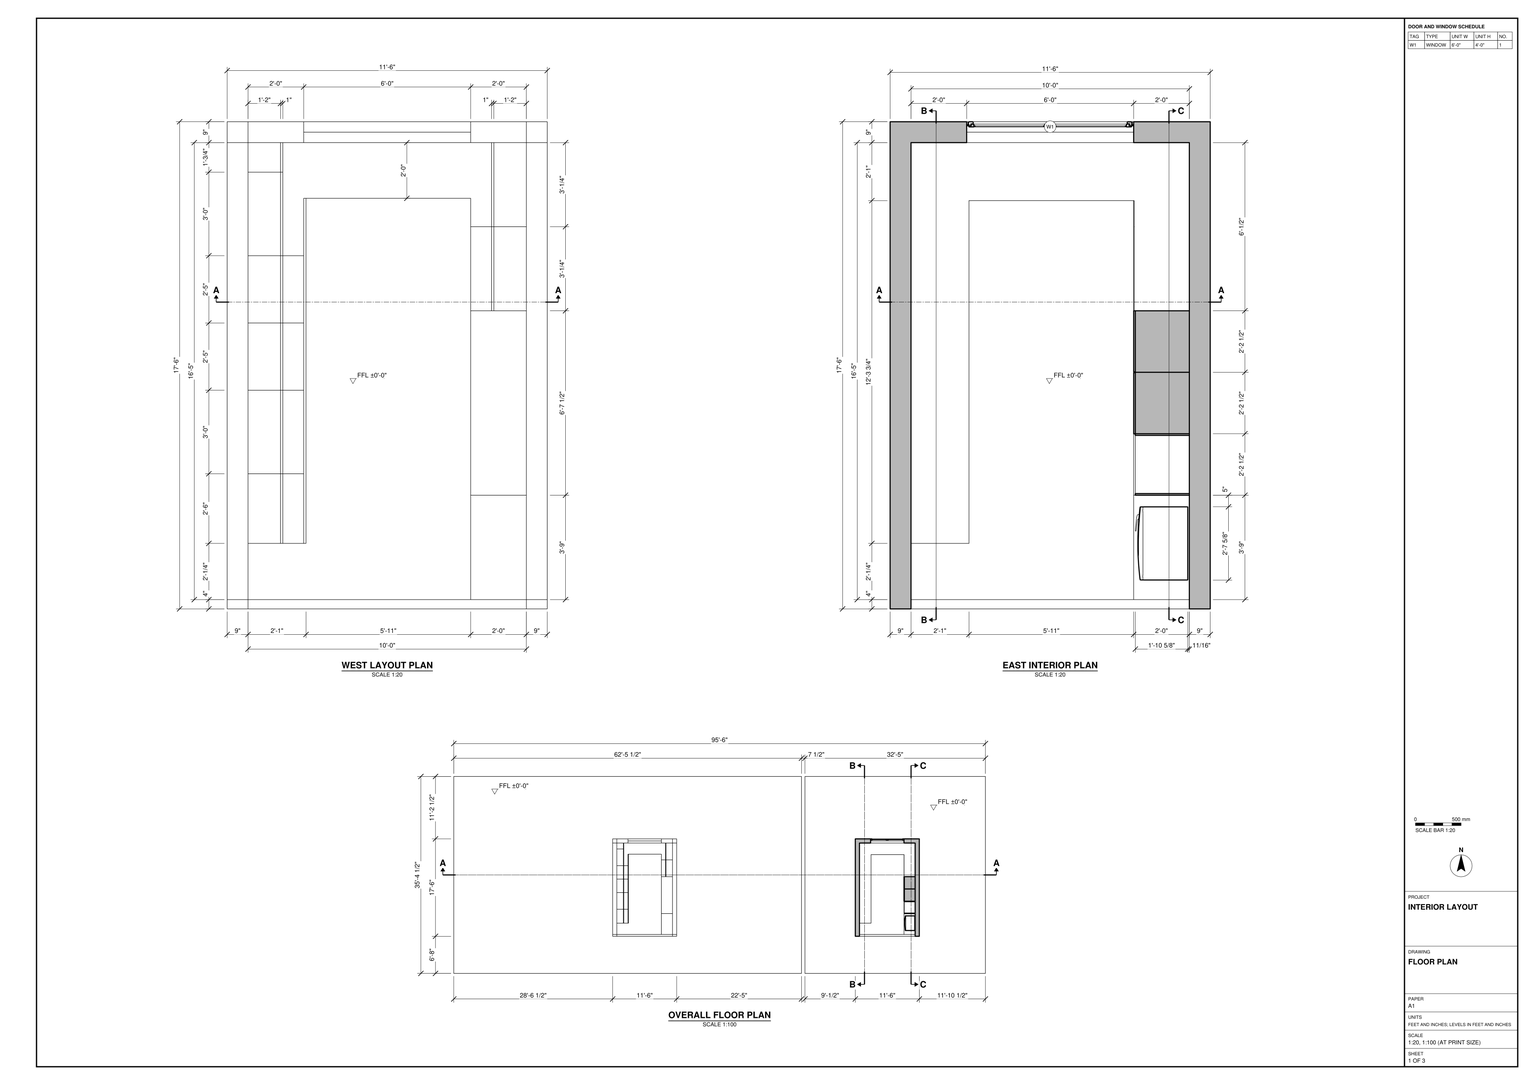
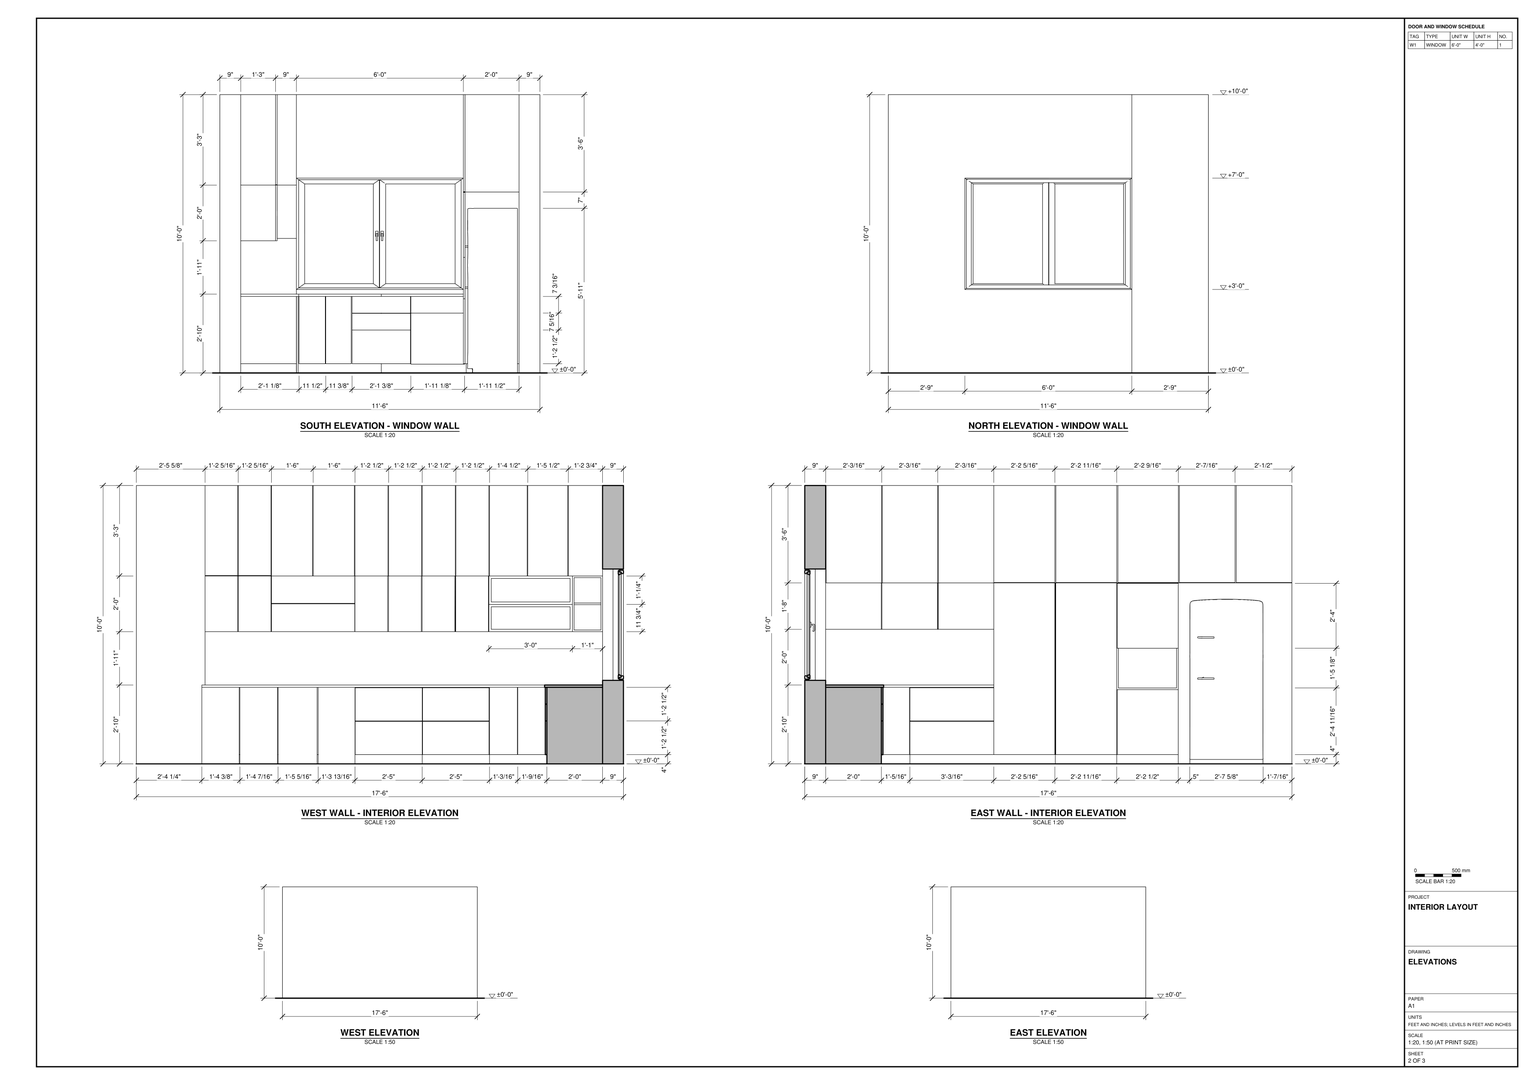
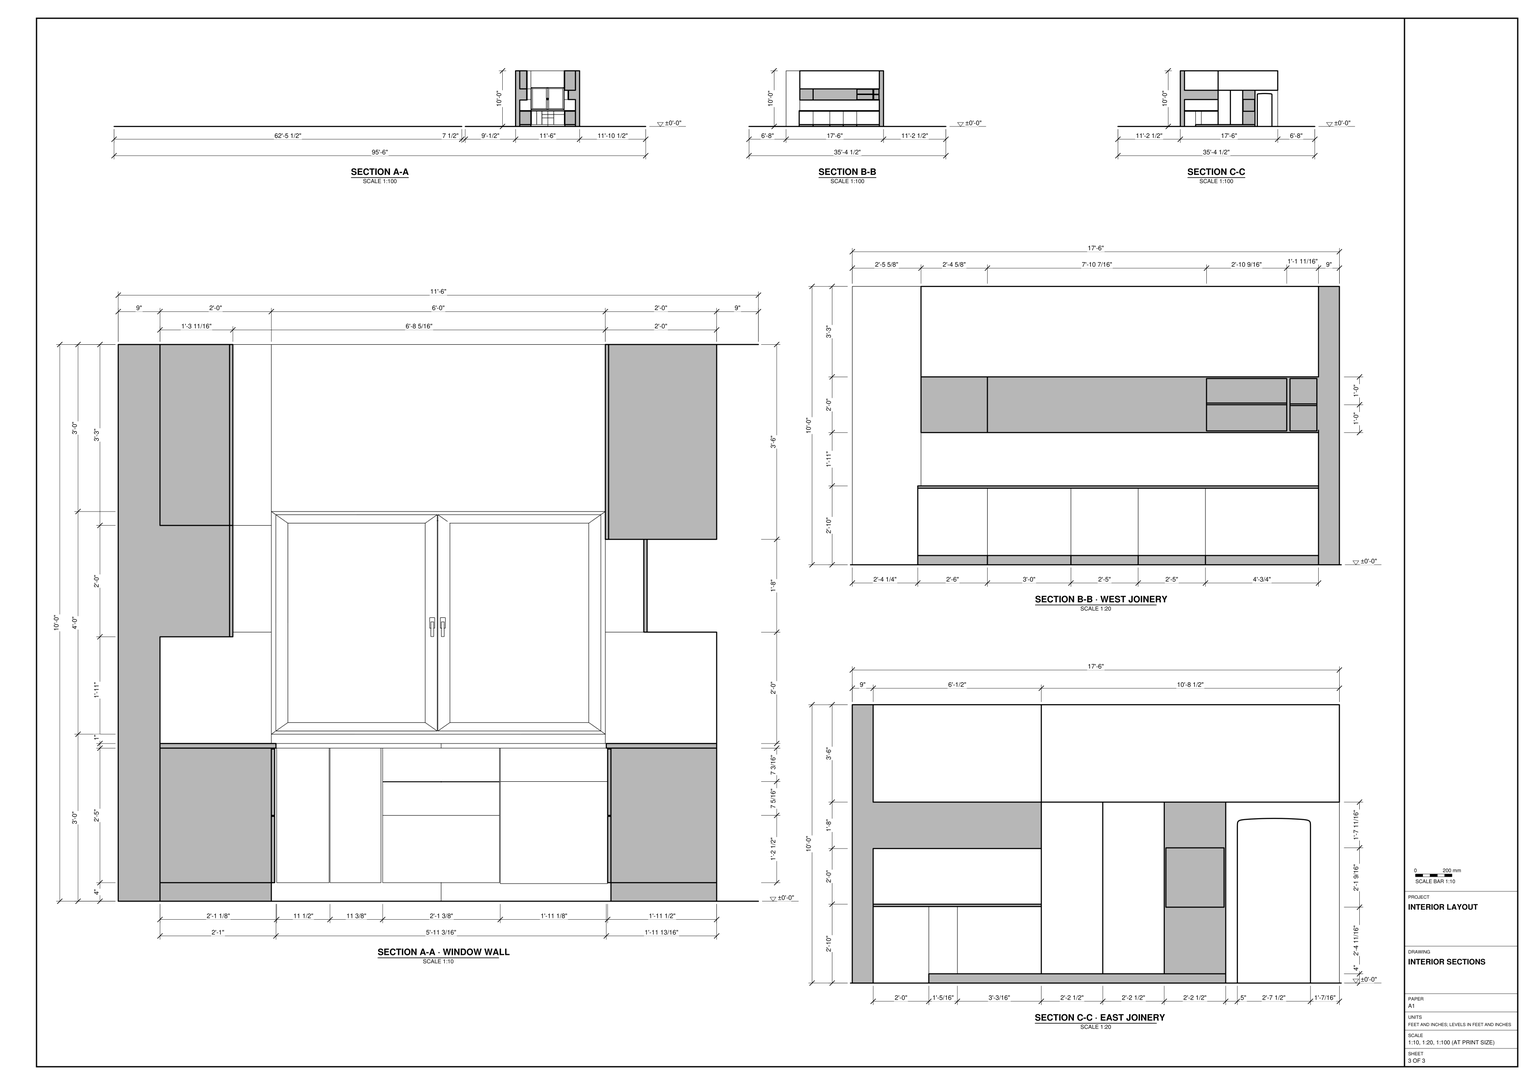
Build one SketchUp model from task_files/diagram_01.pdf. Work in feet and inches. The overall model measures 95'-6" along X, 35'-4 1/2" along Y and 10'-0" high, with a single finished floor level at ±0'-0".

Use the overall floor plan to position the two rectangular floor areas and the gap between them. Show the west layout as a flat plan with the wall outlines, cabinet divisions and central aisle. On the east floor area, build the corresponding kitchen in three dimensions. Its outside footprint is 11'-6" by 17'-6". Build the 9" side walls and window wall, leaving the entrance end open. Center the two-panel window above the counter on the end wall.

Use the interior elevations for the arrangement of cupboard doors, drawers and shelves, and the sections for worktop heights, plinths and cabinet depths. Connect the long west worktop to the base units beneath the window and the shorter east worktop. Continue the east run with tall storage and the refrigerator bay toward the entrance. Decor and loose items, including the refrigerator, may be any suitable library components.

Keep shell elements such as walls and floor areas, and each furniture or joinery piece, in separate groups or components. Use components for repeated parts. Save the completed model as output_files/fitted_kitchen_and_its_companion_plan_layout.skp.

# SketchUp Ruby script. Lengths in inches.
U = 1.inch
M = Sketchup.active_model
def pt(a) = Geom::Point3d.new(a.map { |v| v * U })
def face(e, loops, mat)
  f = e.add_face(loops[0].map { |a| pt(a) })
  loops[1..].each { |l| e.add_face(l.map { |a| pt(a) }).erase! }
  f.material = f.back_material = mat if mat
  f
end
# faces: each face lists its corners as indices into pts; further lists are holes
def faces(e, pts, list, mat = nil) = list.each { |f| face(e, (f[0].is_a?(Array) ? f : [f]).map { |l| l.map { |i| pts[i] } }, mat) }
# xy, xz, yz: faces in a plane at the given z, y or x. An outline is a flat list of corners, or four numbers for a rectangle; further outlines are holes
def ring(l) = l.size == 4 ? [[l[0], l[1]], [l[2], l[1]], [l[2], l[3]], [l[0], l[3]]] : l.each_slice(2).to_a
def flat(e, list, mat, &to3) = list.each { |f| face(e, (f[0].is_a?(Array) ? f : [f]).map { |l| ring(l).map { |u, v| to3.(u, v) } }, mat) }
def xy(e, z, list, mat = nil) = flat(e, list, mat) { |x, y| [x, y, z] }
def xz(e, y, list, mat = nil) = flat(e, list, mat) { |x, z| [x, y, z] }
def yz(e, x, list, mat = nil) = flat(e, list, mat) { |y, z| [x, y, z] }
def lines(e, pts, list) = list.each { |a, b| e.add_line(pt(pts[a]), pt(pts[b])) }
# prism: a flat outline (further loops are holes) pulled along v
def prism(e, loops, v, mat = nil)
  f = face(e, loops, mat); d = Geom::Vector3d.new(v.map { |x| x * U })
  f.pushpull(f.normal.samedirection?(d) ? d.length : -d.length)
end
def box(e, o, s, mat = nil) = prism(e, [[o, [o[0] + s[0], o[1], o[2]], [o[0] + s[0], o[1] + s[1], o[2]], [o[0], o[1] + s[1], o[2]]]], [0, 0, s[2]], mat)
def at(x, y, z, deg = 0) = Geom::Transformation.translation(pt([x, y, z])) * Geom::Transformation.rotation(ORIGIN, Z_AXIS, deg.degrees)
def axes(o, x, y, z) = Geom::Transformation.new([*x, 0, *y, 0, *z, 0, *pt(o).to_a, 1])
def part(name) = M.definitions.add(name)
# library, detail: a bought-in or finely detailed component or shape, given as its bounding box
def library(name, o, s) = part(name).tap { |d| box(d.entities, o, s) }
def detail(e, o, s) = box(e.add_group.entities, o, s)
def put(e, d, t, mat = nil) = e.add_instance(d, t).tap { |i| i.material = mat if mat }
def group(e, t, mat = nil) = e.add_group.tap { |g| g.transformation = t; g.material = mat if mat }.entities
root = M.entities
M.materials.add("Heather_Band").color = [201, 178, 162]
M.materials.add("[Basic Tile]").color = [203, 206, 202]
M.materials.add("[Color B01]").color = [255, 216, 204]
M.materials.add("[Color M00]").color = [255, 255, 255]
M.materials.add("[Marble Carrara Gold Floor Tile]").color = [225, 223, 217]
M.materials.add("[Translucent Glass Gray]").color = [128, 128, 128]
M.materials["[Translucent Glass Gray]"].alpha = 0.5
c1 = library("Fridge 143 008",[-15.8,-16.72,0],[31.6,33.44,70.99])
c2 = library("Window 46-10",[-43.56,-2.12,0],[87.13,4.27,82.67])
c3 = part("Group\#45")
box(c3.entities,[0,0,0],[0.71,23.97,42])
c4 = part("Group\#46")
box(c4.entities,[0,0,0],[0.71,23.97,20])
c5 = part("Group\#8")
box(c5.entities,[0,2.3,0],[0.71,24,41.84])
c6 = part("Group\#27")
box(c6.entities,[0,-6.33,-14.7],[0.71,78.11,14.7])
c7 = part("Group\#51")
box(c7.entities,[0,0.2,0],[0.71,26.3,28])
c8 = part("Group\#23")
prism(c8.entities,[[[24,36,0],[24,0,0],[12.5,0,0],[12.5,36,0]],[[23,35,0],[13.5,35,0],[13.5,1,0],[23,1,0]]],[0,0,0.71])
g1 = group(c8.entities,at(13.5,1,0.6875))
box(g1,[0,0,0],[9.5,34,0.02],"[Translucent Glass Gray]")
c9 = part("Group\#44")
box(c9.entities,[0,0,0],[0.71,14.12,24])
xy(root,0,[[[0,0,749.5,424.5],[342.5,80,480.5,290]],[[757,0,1146,424.5],[865.5,80,1003.5,290]],[342.5,80,351.5,84],[351.5,80,471.5,84],[471.5,80,480.5,84],
  [874.5,80,994.5,84],[342.5,84,351.5,281],[351.5,84,447.5,84,447.5,257,376.5,257,376.5,108.23,351.5,108.23],[447.5,84,471.5,129],[471.5,84,480.5,281],
  [874.5,84,970.5,84,970.5,257,899.5,257,899.5,108.23,874.5,108.23],[970.5,84,994.5,129],[351.5,108.23,365.5,138.25],[365.5,108.23,366.5,138.25],[366.5,108.23,375.5,138.25],
  [375.5,108.23,376.5,257],[874.5,108.23,898.5,138.25],[898.5,108.23,899.5,257],[447.5,129,471.5,208.5],[970.5,129,994.5,155.5],
  [351.5,138.25,365.5,174.25],[365.5,138.25,366.5,174.25],[366.5,138.25,375.5,174.25],[874.5,138.25,898.5,174.25],[970.5,155.5,994.5,182],
  [351.5,174.25,365.5,203.25],[365.5,174.25,366.5,203.25],[366.5,174.25,375.5,203.25],[874.5,174.25,898.5,203.25],[970.5,182,994.5,208.5],
  [351.5,203.25,365.5,232.25],[365.5,203.25,366.5,232.25],[366.5,203.25,375.5,232.25],[874.5,203.25,898.5,232.25],[447.5,208.5,456.5,244.75],
  [456.5,208.5,457.5,244.75],[457.5,208.5,471.5,244.75],[970.5,208.5,994.5,244.75],[351.5,232.25,365.5,268.25],[365.5,232.25,366.5,268.25],
  [366.5,232.25,375.5,232.25,375.5,257,447.5,257,447.5,244.75,456.5,244.75,456.5,281,366.5,281],[874.5,232.25,898.5,232.25,898.5,257,970.5,257,970.5,244.75,994.5,244.75,994.5,281,874.5,281],[456.5,244.75,457.5,281],[457.5,244.75,471.5,281],[351.5,268.25,365.5,281],
  [365.5,268.25,366.5,281],[342.5,281,351.5,290],[351.5,281,375.5,290],[375.5,281,447.5,285.5],[447.5,281,471.5,290],
  [471.5,281,480.5,290],[898.5,281,970.5,285.5],[375.5,285.5,447.5,290],[898.5,285.5,970.5,290]])
put(root,c1,axes([982.51,108.22,0],[0,-1,0],[0.67589,0,0],[0,0,1]))
put(root,c2,axes([934.5,287.85,36],[0.82635,0,0],[0,1,0],[0,0,0.58062]))
g2 = group(root,at(970.5,80,0),"[Basic Tile]")
xy(g2,0,[[24,0,24,201,-72,201,-72,210,33,210,33,0]],"[Color M00]")
xy(g2,36,[[-72,201,0,205.5],[-72,205.5,0,210]],"[Color M00]")
xy(g2,58,[[9,128.5,24,201]],"[Color M00]")
xy(g2,78,[[9,128.5,24,201]],"[Color M00]")
xy(g2,84,[[-72,201,0,205.5],[-72,205.5,0,210]],"[Color M00]")
xy(g2,120,[[24,0,33,0,33,210,-72,210,-72,201,24,201]],"[Color M00]")
xz(g2,0,[[24,0,33,120]],"[Color M00]")
xz(g2,128.5,[[9,58,24,78]],"[Color M00]")
xz(g2,201,[[-72,0,24,0,24,34,0,34,0,36,-72,36],[0,34,24,58]],"[Basic Tile]")
xz(g2,201,[[-96,34,-72,58],[0,58,9,58,9,78,24,78,24,120,-72,120,-72,84,0,84]],"[Color M00]")
xz(g2,210,[[-72,0,-72,36,0,36,0,84,-72,84,-72,120,33,120,33,0]],"[Color M00]")
yz(g2,-72,[[201,0,210,36],[201,84,210,120]],"[Color M00]")
yz(g2,0,[[201,36,205.5,84],[205.5,36,210,84]],"[Color M00]")
yz(g2,9,[[128.5,58,152.67,78],[152.67,58,201,78]],"[Color M00]")
yz(g2,24,[[128.5,34,201,58]],"[Basic Tile]")
yz(g2,24,[[0,0,0,78,128.5,78,128.5,34,201,34,201,0]],"[Color B01]")
yz(g2,24,[[0,78,128.5,120],[128.5,78,201,120]],"[Color M00]")
yz(g2,33,[[0,0,210,120]],"[Color M00]")
g3 = group(g2,at(0,0,78))
xy(g3,0,[[0.71,0,24,128.5],[0.71,128.5,24,201]])
xy(g3,42,[[0.71,0,24,128.5],[0.71,128.5,24,201]],"Heather_Band")
xz(g3,0,[[0.71,0,24,42]])
xz(g3,128.5,[[0.71,0,24,42]])
xz(g3,201,[[0.71,0,24,42]])
yz(g3,0.71,[[0,0,128.5,42],[128.5,0,152.67,42],[152.67,0,176.83,42],[176.83,0,201,42]])
yz(g3,24,[[0,0,128.5,42],[128.5,0,201,42]])
put(g3,c3,at(0,128.5,0),"Heather_Band")
put(g3,c3,at(0,152.67,0),"Heather_Band")
put(g3,c3,at(0,176.83,0),"Heather_Band")
put(g2,c4,at(8.29,128.5,58),"[Color B01]")
put(g2,c4,at(8.29,152.77,58),"[Color B01]")
put(g2,c4,at(8.29,177.03,58),"[Color B01]")
g4 = group(root,at(970.5,129,0),"[Marble Carrara Gold Floor Tile]")
xy(g4,0,[[-96,-20.77,-72,9.25],[0,0,1.21,26.5],[-96,9.25,-72,45.25],[0,26.5,1.21,53],[-96,45.25,-72,74.25],
  [0,53,1.21,79.5],[-96,74.25,-72,103.25],[1.21,79.5,24,128],[-96,103.25,-72,152],[-72,128,24,152]])
xy(g4,4,[[-96,-20.77,-72,9.25],[0.71,0,1.21,26.5],[1.21,0,24,26.5],[-96,9.25,-72,45.25],[0.71,26.5,1.21,53],
  [1.21,26.5,24,53],[-96,45.25,-72,74.25],[0.71,53,1.21,79.5],[1.21,53,24,79.5],[-96,74.25,-72,103.25],
  [1.21,79.5,24,115.67],[-96,103.25,-72,152],[1.21,115.67,24,128]])
xy(g4,32.71,[[0.71,0.71,24,25.79]],"[Color B01]")
xy(g4,33,[[-96,-20.77,-72,-20.77,-72,128,1.21,128,1.21,79.5,24,79.5,24,152,-96,152]])
xy(g4,58.29,[[0.71,0.71,24,25.79]])
xy(g4,78,[[0.71,0,24,26.5],[0.71,26.5,24,53],[0.71,53,24,79.5]])
xz(g4,-20.77,[[-96,0,-72,4],[-96,4,-72,33]],"Heather_Band")
xz(g4,0,[[1.21,0,24,4]])
xz(g4,0,[[0.71,4,24,78]],"[Color B01]")
xz(g4,0.71,[[0.71,32.71,24,58.29]],"[Color B01]")
xz(g4,9.25,[[-96,0,-72,4]])
xz(g4,25.79,[[0.71,32.71,24,58.29]],"[Color B01]")
xz(g4,26.5,[[0.71,4,24,78]])
xz(g4,45.25,[[-96,0,-72,4]])
xz(g4,53,[[0.71,4,24,78]])
xz(g4,74.25,[[-96,0,-72,4]])
xz(g4,79.5,[[0.71,4,0.71,78,24,78,24,33,1.21,33,1.21,4],[1.21,4,24,33]])
xz(g4,103.25,[[-96,0,-72,4]])
xz(g4,128,[[1.21,0,24,4]])
xz(g4,128,[[-72,0,-35.4,33],[-35.4,0,1.21,33]],"Heather_Band")
xz(g4,152,[[-96,0,-72,4],[-72,0,24,33],[-96,4,-72,33]])
yz(g4,-96,[[-20.77,0,9.25,4],[9.25,0,45.25,4],[45.25,0,74.25,4],[74.25,0,103.25,4],[103.25,0,152,4],
  [-20.77,4,9.25,33],[9.25,4,45.25,33],[45.25,4,74.25,33],[74.25,4,103.25,33],[103.25,4,152,33]])
yz(g4,-72,[[128,0,152,4],[45.25,4,74.25,33],[74.25,4,103.25,33],[103.25,4,128,33]])
yz(g4,-72,[[-20.77,0,9.25,4],[9.25,0,45.25,4],[45.25,0,74.25,4],[74.25,0,103.25,4],[103.25,0,128,4],
  [-20.77,4,9.25,33],[9.25,4,45.25,33]],"Heather_Band")
yz(g4,0.71,[[0,4,26.5,32],[26.5,4,53,78],[53,4,79.5,78],[0,59,26.5,78]])
yz(g4,0.71,[[[0,32,26.5,59],[0.71,32.71,25.79,58.29]]],"[Color B01]")
yz(g4,1.21,[[79.5,4,115.67,18.5],[115.67,4,128,33],[79.5,18.5,115.67,33]])
yz(g4,1.21,[[0,0,26.5,4],[26.5,0,53,4],[53,0,115.67,4],[115.67,0,128,4]],"[Color B01]")
yz(g4,24,[[0,0,26.5,4],[26.5,0,53,4],[53,0,128,4],[128,0,152,33],[[0,4,26.5,78],[0.71,32.71,25.79,58.29]],
  [26.5,4,53,78],[53,4,79.5,78],[79.5,4,115.67,33],[115.67,4,128,33]])
g5 = group(g4,at(0,53.2,4))
xy(g5,0,[[0,0,0.71,26.3]])
xy(g5,74,[[0,0,0.71,26.3]])
xz(g5,0,[[0,0,0.71,74]])
xz(g5,26.3,[[0,0,0.71,74]])
yz(g5,0,[[0,0,26.3,74]],"[Color B01]")
yz(g5,0.71,[[0,0,26.3,74]])
g6 = group(g4,at(0,26.5,4),"[Color B01]")
xy(g6,0,[[0,0,0.71,26.3]])
xy(g6,74,[[0,0,0.71,26.3]])
xz(g6,0,[[0,0,0.71,74]])
xz(g6,26.3,[[0,0,0.71,74]])
yz(g6,0,[[0,0,26.3,74]],"[Color B01]")
yz(g6,0.71,[[0,0,26.3,74]])
g7 = group(g4,at(0,53.2,78.16),"Heather_Band")
box(g7,[0,0,0],[0.71,26.3,41.84])
g8 = group(g4,at(0,26.45,78.16),"Heather_Band")
box(g8,[0,0.05,0],[0.71,26.25,41.84])
g9 = group(g4,at(0,-0.3,78.16),"Heather_Band")
box(g9,[0,0.24,0],[0.71,26.06,41.84])
put(g4,c5,at(0,-26.8,78.16),"Heather_Band")
put(g4,c5,at(0,-51.3,78.16),"Heather_Band")
g10 = group(g4,at(0.5,79.5,4),"Heather_Band")
box(g10,[0,0,0],[0.71,36.17,14.3])
g11 = group(g4,at(0.5,79.5,18.5),"Heather_Band")
box(g11,[0,0,0],[0.71,36.17,14.3])
g12 = group(g4,at(0.5,115.83,18.7),"Heather_Band")
box(g12,[0,0,-14.7],[0.71,11.66,29])
g13 = group(g4,at(0.5,127.29,33),"Heather_Band")
box(g13,[-23.14,0,-7.2],[23.14,0.71,7.2])
g14 = group(g4,at(-35.48,127.29,17.5),"Heather_Band")
box(g14,[-12.52,0,-13.5],[25.18,0.71,14.5])
g15 = group(g4,at(-71.29,127.3125,17.5),"Heather_Band")
box(g15,[-0.71,-11.89,-13.5],[0.71,12.03,29])
g16 = group(g4,at(-71.29,115.14,17.5),"Heather_Band")
box(g16,[-0.71,-11.89,-13.5],[0.71,12.03,29])
g17 = group(g4,at(0.5,127.29,18.3),"Heather_Band")
box(g17,[-23.14,0,-14.5],[23.14,0.71,29.2])
g18 = group(g4,at(-71.29,102.92,17.5),"Heather_Band")
box(g18,[-0.71,-28.51,-13.5],[0.71,28.65,14.3])
g19 = group(g4,at(-71.2,57.23,17.5),"Heather_Band")
box(g19,[-0.71,-11.89,-13.5],[0.71,28.91,14.3])
g20 = group(g4,at(-71.29,102.92,32),"Heather_Band")
box(g20,[-0.71,-28.51,-13.5],[0.71,28.65,14.3])
g21 = group(g4,at(-71.2,57.23,32),"Heather_Band")
box(g21,[-0.71,-11.89,-13.5],[0.71,28.91,14.3])
put(g4,c6,axes([-24.86,127.29,33],[0,1,0],[-0.32242,0,0],[0,0,0.4899]),"Heather_Band")
put(g4,c6,axes([-24.86,127.29,25.7],[0,1,0],[-0.32242,0,0],[0,0,0.4899]),"Heather_Band")
g22 = group(g4,at(-48.51,127.29,17.5),"Heather_Band")
box(g22,[-10.84,0,-13.5],[10.98,0.71,29])
g23 = group(g4,at(-61.01,127.29,17.5),"Heather_Band")
box(g23,[-9.84,0,-13.5],[11.3,0.71,29])
g24 = group(g4,at(-96,-20.77,33))
prism(g24,[[[60.6,147.77,0],[25,147.77,0],[25,0,0],[0,0,0],[0,30.02,0],[0,66.02,0],[0,95.02,0],[0,124.02,0],[0,172.77,0],[24,172.77,0],[120,172.77,0],[120,148.77,0],[120,136.44,0],[120,100.27,0],[96.21,100.27,0],[96.21,147.77,0]]],[0,0,1])
g25 = group(g4,at(-71.24,23.98,17.5),"Heather_Band")
box(g25,[-0.71,-11.89,-17.5],[0.71,16.85,33])
g26 = group(g4,at(-71.29,42.79,17.5),"Heather_Band")
box(g26,[-0.71,-13.39,-17.5],[0.71,15.85,33])
g27 = group(g4,at(-71.24,6.94,17.5),"Heather_Band")
box(g27,[-0.71,-11.3125,-17.5],[0.71,16.27,33])
g28 = group(g4,at(-71.24,-10.08,17.5),"Heather_Band")
box(g28,[-0.71,-10.6875,-17.5],[0.71,16.11,33])
put(g4,c7,at(0,-0.2,4),"[Color B01]")
put(g4,c7,at(0,-0.2,49.83),"[Color B01]")
g29 = group(root,at(865.5,80,0))
xy(g29,0,[[0,0,0,210,33,210,33,201,9,201,9,0]])
xy(g29,57,[[9,29.62,24,58.25],[9,58.25,24,94.25],[9,94.25,24,152],[9,152,24,188],[9,188,23.5,201]])
xy(g29,57.71,[[9.71,152.71,24,187.29],[9.71,188.71,23.5,200.29]])
xy(g29,80.29,[[9.71,152.71,24,187.29],[9.71,188.71,23.5,200.29]])
xy(g29,81,[[9,29.62,24,58.25],[9,58.25,9,201,23.5,201,23.5,188,24,188,24,58.25],[23.5,188,24,201]])
xy(g29,120,[[0,0,9,0,9,201,33,201,33,210,0,210],[9,29.62,24,201]])
xz(g29,0,[[0,0,9,120]])
xz(g29,29.62,[[9,57,24,81],[9,81,24,120]])
xz(g29,58.25,[[9,57,24,81]])
xz(g29,152.71,[[9.71,57.71,24,80.29]])
xz(g29,187.29,[[9.71,57.71,24,80.29]])
xz(g29,188,[[23.5,57,24,81]])
xz(g29,188.71,[[9.71,57.71,23.5,80.29]])
xz(g29,200.29,[[9.71,57.71,23.5,80.29]])
xz(g29,201,[[9,0,33,0,33,81,23.5,81,23.5,57,9,57],[9,81,24,120],[24,81,33,120]])
xz(g29,210,[[0,0,33,120]])
yz(g29,0,[[0,0,210,120]])
yz(g29,9,[[0,0,201,0,201,34,29.62,34,29.62,120,0,120],[29.62,57,58.25,81],[29.62,81,201,120]])
yz(g29,9,[[29.62,34,201,57]],"[Basic Tile]")
yz(g29,9.71,[[152.71,57.71,187.29,80.29],[188.71,57.71,200.29,80.29]])
yz(g29,23.5,[[[188,57,201,81],[188.71,57.71,200.29,80.29]]])
yz(g29,24,[[29.62,57,43.94,81],[43.94,57,58.25,81],[58.25,57,94.25,81],[137.5,57,152,57,152,81,137.5625,81],[[152,57,188,81],[152.71,57.71,187.29,80.29]],
  [29.62,81,58.25,120],[58.25,81,201,120]])
yz(g29,24,[[94.25,57,137.5,57,137.5625,81,94.25,81]],"[Color B01]")
yz(g29,33,[[201,0,205.5,120],[205.5,0,210,120]])
g30 = group(g29,at(24,140.45,81),"Heather_Band")
box(g30,[0,-2.69,0],[0.71,14.24,39])
g31 = group(g29,at(9.71,188.71,68.65))
box(g31,[0,0,0],[13.79,11.58,0.71])
g32 = group(g29,at(9.71,152.71,69))
box(g32,[0,0,0],[13.79,34.58,0.71])
put(g29,c8,axes([24,152,81.48],[0,0,-1.02],[0,1,0],[1,0,0]))
put(g29,c8,axes([24,152,94.34],[0,0,-1.06696],[0,1,0],[1,0,0]))
g33 = group(g29,at(24,76.17,57),"[Color B01]")
box(g33,[0,-17.92,0],[0.71,35.92,12])
g34 = group(g29,at(24,76.17,69.2),"[Color B01]")
box(g34,[0,-17.92,0],[0.71,35.92,11.8])
g35 = group(g29,at(24,125.95,81),"Heather_Band")
box(g35,[0,-2.69,0],[0.71,14.24,39])
g36 = group(g29,at(24,111.44,81),"Heather_Band")
box(g36,[0,-2.69,0],[0.71,14.24,39])
g37 = group(g29,at(24,96.94,81),"Heather_Band")
box(g37,[0,-2.69,0],[0.71,14.24,39])
g38 = group(g29,at(24,154.95,81),"Heather_Band")
box(g38,[0,-2.69,0],[0.71,16.24,39])
g39 = group(g29,at(24,173.95,81),"Heather_Band")
box(g39,[0,-5.19,0],[0.71,17.24,39])
g40 = group(g29,at(24,188.95,81),"Heather_Band")
box(g40,[0,-2.69,0],[0.71,14.74,39])
g41 = group(g29,at(24,82.4375,81),"Heather_Band")
box(g41,[0,-6.19,0],[0.71,17.74,39])
g42 = group(g29,at(24,63.94,81),"Heather_Band")
box(g42,[0,-5.69,0],[0.71,17.74,39])
put(g29,c9,at(24,29.62,57),"[Color B01]")
put(g29,c9,at(24,43.94,57),"[Color B01]")
g43 = group(g29,at(24,29.62,96),"Heather_Band")
box(g43,[0,0,-14.8],[0.71,14.12,38.8])
g44 = group(g29,at(24,43.94,96),"Heather_Band")
box(g44,[0,0,-14.8],[0.71,14.12,38.8])
put(g29,c9,at(24,137.69,57),"[Color B01]")
put(g29,c9,at(24,123.21,57),"[Color B01]")
put(g29,c9,at(24,108.73,57),"[Color B01]")
put(g29,c9,at(24,94.25,57),"[Color B01]")
